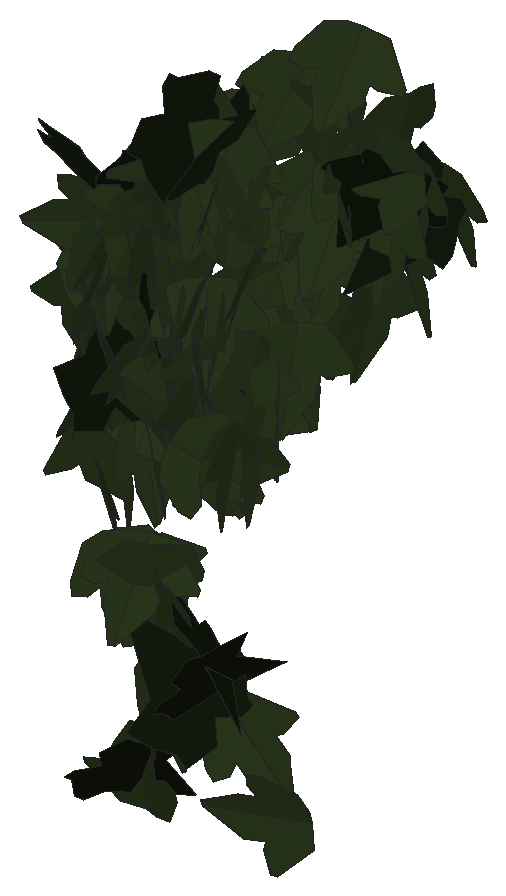
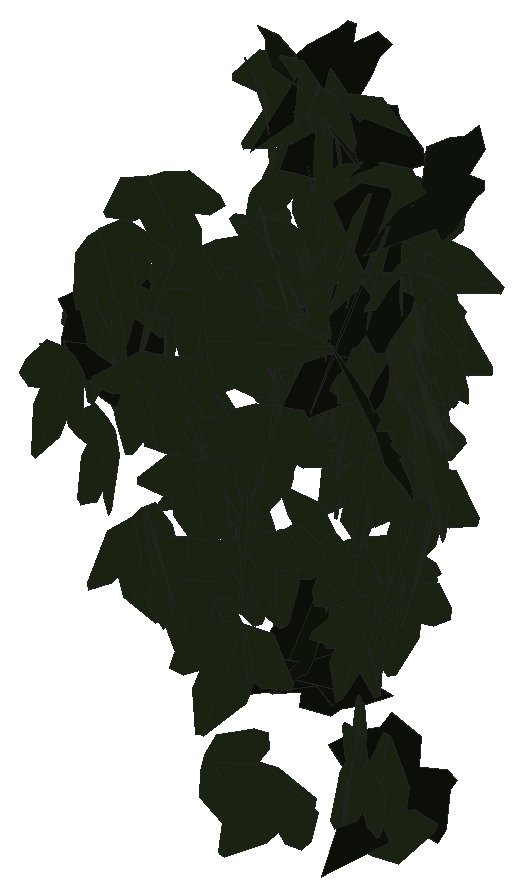
# SketchUp Ruby script. Lengths in inches.
U = 1.inch
M = Sketchup.active_model
def pt(a) = Geom::Point3d.new(a.map { |v| v * U })
def face(e, loops, mat)
  f = e.add_face(loops[0].map { |a| pt(a) })
  loops[1..].each { |l| e.add_face(l.map { |a| pt(a) }).erase! }
  f.material = f.back_material = mat if mat
  f
end
# faces: each face lists its corners as indices into pts; further lists are holes
def faces(e, pts, list, mat = nil) = list.each { |f| face(e, (f[0].is_a?(Array) ? f : [f]).map { |l| l.map { |i| pts[i] } }, mat) }
# xy, xz, yz: faces in a plane at the given z, y or x. An outline is a flat list of corners, or four numbers for a rectangle; further outlines are holes
def ring(l) = l.size == 4 ? [[l[0], l[1]], [l[2], l[1]], [l[2], l[3]], [l[0], l[3]]] : l.each_slice(2).to_a
def flat(e, list, mat, &to3) = list.each { |f| face(e, (f[0].is_a?(Array) ? f : [f]).map { |l| ring(l).map { |u, v| to3.(u, v) } }, mat) }
def xy(e, z, list, mat = nil) = flat(e, list, mat) { |x, y| [x, y, z] }
def xz(e, y, list, mat = nil) = flat(e, list, mat) { |x, z| [x, y, z] }
def yz(e, x, list, mat = nil) = flat(e, list, mat) { |y, z| [x, y, z] }
def lines(e, pts, list) = list.each { |a, b| e.add_line(pt(pts[a]), pt(pts[b])) }
# prism: a flat outline (further loops are holes) pulled along v
def prism(e, loops, v, mat = nil)
  f = face(e, loops, mat); d = Geom::Vector3d.new(v.map { |x| x * U })
  f.pushpull(f.normal.samedirection?(d) ? d.length : -d.length)
end
def box(e, o, s, mat = nil) = prism(e, [[o, [o[0] + s[0], o[1], o[2]], [o[0] + s[0], o[1] + s[1], o[2]], [o[0], o[1] + s[1], o[2]]]], [0, 0, s[2]], mat)
def at(x, y, z, deg = 0) = Geom::Transformation.translation(pt([x, y, z])) * Geom::Transformation.rotation(ORIGIN, Z_AXIS, deg.degrees)
def axes(o, x, y, z) = Geom::Transformation.new([*x, 0, *y, 0, *z, 0, *pt(o).to_a, 1])
def part(name) = M.definitions.add(name)
# library, detail: a bought-in or finely detailed component or shape, given as its bounding box
def library(name, o, s) = part(name).tap { |d| box(d.entities, o, s) }
def detail(e, o, s) = box(e.add_group.entities, o, s)
def put(e, d, t, mat = nil) = e.add_instance(d, t).tap { |i| i.material = mat if mat }
def group(e, t, mat = nil) = e.add_group.tap { |g| g.transformation = t; g.material = mat if mat }.entities
root = M.entities
M.materials.add("efeu1").color = [18, 25, 13]
M.materials.add("efeu2").color = [43, 57, 29]
c1 = part("ivyleaf_9")
p = [[1.54,2.16,1.25],[1.36,2.04,1.19],[-0.21,0.99,0.68],[-0.71,1.11,0.82],[-0.85,0.86,0.67],[-0.8,0.17,0.21],
  [-0.9,-0.01,0.1],[-0.67,-0.16,-0.02],[-0.08,-0.08,-0.05],[-0.03,-0.6,-0.4],[0.65,-0.88,-0.66],[0.83,-0.6,-0.49],
  [1.29,-0.42,-0.43],[1.8125,-0.07,-0.26],[1.21,0.44,0.15]]
faces(c1.entities,p,[[0,1,2,3,4,5,6,7,8,9,10,11,12,13,14]],"efeu1")
c2 = part("ivyleaf_10")
p = [[0,0.5,-0.03],[-0.0625,2.02,-0.43],[-0.19,2.01,-0.46],[-0.54,1.05,-0.29],[-0.52,0.625,-0.18],[-0.83,0.76,-0.28],
  [-1.16,0.64,-0.33],[-1.15,0.33,-0.24],[-0.77,-0.39,0.02],[-0.3,-0.51,0.16],[0.04,-0.48,0.23],[-0.02,2.01,-0.4375],
  [-0.06,2.01,-0.43],[0.04,-0.49,0.23],[0.67,-0.49,0.14],[1.38,0.36,-0.2],[1.375,0.51,-0.24],[0.81,0.65,-0.19],
  [0.62,0.59,-0.15],[0.6,1.09,-0.28],[0.5,1.23,-0.31]]
faces(c2.entities,p,[[0,1,2,3,4,5,6,7,8,9,10],[11,12,0,13,14,15,16,17,18,19,20]],"efeu2")
put(root,c1,axes([28.5,224.64,221.63],[0.47102,-0.15737,-0.05806],[-0.01733,0.12648,-0.48343],[0.16685,0.45742,0.1137]))
put(root,c2,axes([29.86,224.82,220.2],[0.40488,-0.28287,-0.07784],[-0.05263,0.06047,-0.49353],[0.28863,0.40783,0.01919]))
put(root,c2,axes([29.51,224.96,221.18],[-0.30399,-0.33355,0.21525],[-0.06846,-0.22299,-0.44225],[0.39103,-0.29835,0.0899]))
put(root,c2,axes([28.96,224.83,220.77],[0.15244,0.0172,-0.47589],[-0.47541,0.03413,-0.15105],[0.02729,0.49854,0.02676]))
put(root,c2,axes([30.44,224.62,219.81],[-0.21565,0.39061,0.22566],[-0.18174,0.15369,-0.43972],[-0.41288,-0.27167,0.07569]))
put(root,c2,axes([29.75,224.79,220.58],[-0.14398,0.47231,-0.07871],[0.02061,-0.07601,-0.49376],[-0.47838,-0.14542,0.00241]))
put(root,c2,axes([30.32,224.84,221.86],[-0.46236,0.14744,-0.12036],[0.08114,-0.13332,-0.47502],[-0.17217,-0.45879,0.09936]))
put(root,c1,axes([29.22,224.6875,218.73],[-0.21591,-0.302,0.33493],[0.19308,0.27368,0.37124],[-0.40756,0.28965,-0.00156]))
put(root,c2,axes([29.87,224.83,221.91],[-0.35993,-0.3449,-0.03865],[0.07684,-0.02489,-0.49343],[0.33845,-0.36114,0.07093]))
put(root,c2,axes([29.43,224.89,216.83],[0.38309,0.29352,-0.13072],[-0.09704,-0.08823,-0.48249],[-0.30631,0.39505,-0.01064]))
put(root,c1,axes([30.08,224.54,222.55],[0.15728,-0.13643,-0.45459],[-0.14102,0.44384,-0.18199],[0.45319,0.18546,0.10113]))
put(root,c2,axes([28.93,224.86,220.3],[0.2334,-0.44039,-0.03974],[-0.00565,0.04196,-0.4982],[0.44215,0.23301,0.01461]))
put(root,c2,axes([29.92,224.88,221.75],[-0.00922,-0.49985,-0.00831],[-0.00228,0.00835,-0.49993],[0.49991,-0.00918,-0.00243]))
put(root,c2,axes([29.28,224.93,219.24],[0.09109,-0.49047,0.0338],[0.00236,-0.03393,-0.49884],[0.49163,0.09103,-0.00387]))
put(root,c2,axes([30.38,224.92,221.83],[0.34542,0.33796,-0.12832],[-0.09579,-0.08556,-0.48322],[-0.34858,0.35842,0.00564]))
put(root,c2,axes([28.92,224.82,220.49],[0.07314,0.49378,-0.02883],[-0.01014,-0.02764,-0.49913],[-0.49452,0.0736,0.00597]))
put(root,c2,axes([30.56,224.875,222.22],[0.47817,0.1461,0.00346],[-0.00579,0.03077,-0.49902],[-0.14603,0.47719,0.03112]))
put(root,c1,axes([30.62,224.67,222.26],[-0.21297,0.40707,0.19732],[-0.17522,0.12684,-0.45079],[-0.41706,-0.26116,0.08863]))
put(root,c1,axes([29.24,224.53,214.37],[0.32817,0.34815,0.14525],[0.09195,0.11288,-0.47833],[-0.36586,0.34066,0.01006]))
put(root,c2,axes([30.58,224.99,218.59],[0.18188,-0.45439,0.10222],[0.10643,-0.06629,-0.48402],[0.45342,0.19783,0.07261]))
put(root,c2,axes([29.58,224.89,216.84],[-0.36258,-0.3396,0.0566],[-0.04507,-0.03466,-0.49676],[0.34132,-0.36533,-0.00548]))
put(root,c2,axes([29.05,224.73,219.42],[-0.35572,0.30882,0.16761],[-0.14985,0.0824,-0.46985],[-0.31782,-0.3845,0.03393]))
put(root,c2,axes([30.3,224.86,220.24],[0.42861,0.2521,0.05235],[0.03483,0.04396,-0.49684],[-0.25512,0.42955,0.02012]))
put(root,c2,axes([30.29,224.99,220.06],[0.40896,-0.25464,0.13382],[0.12416,-0.05356,-0.48137],[0.25948,0.42695,0.01942]))
put(root,c2,axes([28.87,225,220.33],[0.15952,-0.46639,0.08388],[0.04466,-0.07332,-0.49258],[0.47176,0.16464,0.01826]))
put(root,c2,axes([29.44,224.84,221.26],[-0.48057,-0.1347,0.0302],[-0.02883,-0.00905,-0.49909],[0.135,-0.48143,0.00093]))
put(root,c2,axes([30.36,225.02,219.4],[0.26041,-0.1776,-0.38813],[0.32126,-0.21781,0.3152],[-0.28104,-0.41354,0.00067]))
put(root,c2,axes([28.71,224.875,219.77],[-0.48333,-0.11894,0.04735],[-0.04415,-0.01871,-0.4977],[0.12016,-0.48529,0.00758]))
put(root,c1,axes([29.77,224.77,221.82],[0.18253,0.42089,-0.19883],[-0.08547,-0.17964,-0.45872],[-0.45758,0.20145,0.00637]))
put(root,c2,axes([30.37,224.96,221.7],[0.26776,-0.4187,-0.05477],[-0.02497,0.04904,-0.49696],[0.42152,0.26887,0.00535]))
put(root,c2,axes([30.3,224.625,218.47],[0.09526,0.29277,0.39396],[0.13006,0.37192,-0.30784],[-0.4733,0.16113,-0.00529]))
put(root,c2,axes([29.79,224.92,219.03],[-0.24499,0.42846,-0.07999],[0.00105,-0.09118,-0.49161],[-0.43587,-0.24105,0.04377]))
put(root,c1,axes([30.27,225.01,215.16],[-0.37535,-0.32362,-0.06625],[-0.0449,-0.04936,0.49553],[-0.32726,0.37794,0.00799]))
put(root,c2,axes([29.33,225.01,213.85],[-0.49988,0.00402,0.01023],[0.01019,-0.00493,0.49987],[0.00412,0.49996,0.00485]))
put(root,c2,axes([30.21,224.91,221.34],[-0.47942,-0.12458,0.06807],[-0.06848,-0.00704,-0.49524],[0.12436,-0.48418,-0.01031]))
put(root,c2,axes([28.68,224.99,218.59],[0.13114,-0.48104,-0.03747],[-0.00739,0.03682,-0.49859],[0.48244,0.13132,0.00255]))
put(root,c2,axes([30.47,224.98,219.66],[-0.23989,-0.43853,-0.01186],[0.00641,0.01002,-0.49986],[0.43865,-0.23997,0.00082]))
put(root,c1,axes([30.28,224.57,215.67],[0.21704,0.29037,0.34435],[0.18781,0.28909,-0.36215],[-0.40942,0.28655,0.01642]))
put(root,c2,axes([30.01,225.06,218.98],[0.08369,-0.4923,0.02514],[-0.00173,-0.02579,-0.49933],[0.49294,0.08349,-0.00602]))
put(root,c2,axes([28.92,225.04,219.82],[0.07813,-0.49384,0.00433],[0.00065,-0.00428,-0.49998],[0.49386,0.07813,-0.00002]))
put(root,c2,axes([29.57,224.9,221.23],[-0.29952,-0.35578,-0.18359],[0.13765,0.12378,-0.46447],[0.37595,-0.32878,0.0238]))
put(root,c1,axes([29.95,225.23,215.98],[0.20827,-0.38455,0.24238],[0.12913,-0.20557,-0.43711],[0.43583,0.24467,0.01369]))
put(root,c2,axes([28.49,225.04,219.85],[0.43149,-0.23739,0.0864],[0.12455,0.05112,-0.48153],[0.21979,0.43707,0.10325]))
put(root,c2,axes([28.51,225.2,219.41],[0.26146,-0.3783,0.19628],[0.11171,-0.1614,-0.45986],[0.41129,0.28432,0.00012]))
put(root,c2,axes([28.85,225.03,220.05],[0.26042,-0.41768,-0.08788],[-0.049,0.07301,-0.49221],[0.424,0.26498,-0.0029]))
put(root,c2,axes([28.71,224.93,220.2],[-0.48793,0.09989,0.04415],[-0.04199,0.01498,-0.49801],[-0.10082,-0.48969,-0.00622]))
put(root,c2,axes([29.93,225.07,219.88],[0.03164,-0.49898,-0.00439],[-0.01479,0.00346,-0.49977],[0.49878,0.03175,-0.01454]))
put(root,c2,axes([29.38,224.86,218.93],[-0.30313,-0.20771,-0.33907],[0.28343,0.18617,-0.36743],[0.27889,-0.41497,0.00488]))
put(root,c2,axes([29.86,224.92,220.4375],[-0.09439,0.48776,0.05641],[-0.00979,0.05556,-0.49681],[-0.49091,-0.09489,-0.00094]))
put(root,c2,axes([29.21,225.11,219.68],[-0.19374,-0.07213,0.45526],[-0.43067,-0.14767,-0.20667],[0.16427,-0.47222,-0.00491]))
put(root,c2,axes([28.78,225.17,219.78],[0.10086,-0.48315,0.07996],[0.00636,-0.08034,-0.49346],[0.48968,0.10056,-0.01006]))
put(root,c2,axes([29.7,225.08,218.61],[-0.29428,0.3865,-0.1184],[-0.00837,-0.15225,-0.47618],[-0.40414,-0.27828,0.09607]))
put(root,c2,axes([29.43,225.06,220.03],[-0.46218,0.06864,-0.17799],[0.16556,-0.08745,-0.46362],[-0.09477,-0.48749,0.05811]))
put(root,c2,axes([29.67,224.95,216.42],[-0.38508,0.05095,0.31483],[-0.30998,0.05631,-0.38825],[-0.07502,-0.4942,-0.01178]))
put(root,c2,axes([29.03,225.03,216.66],[0.3296,0.37326,0.04519],[0.03317,0.031,-0.49793],[-0.37452,0.33124,-0.00433]))
put(root,c2,axes([29.91,225.11,219.95],[-0.06857,0.48267,-0.11101],[-0.03777,-0.11684,-0.48469],[-0.49383,-0.05808,0.05248]))
put(root,c2,axes([30.12,225.09,220.25],[0.16913,-0.46492,-0.07241],[0.00618,0.07914,-0.49366],[0.47048,0.16609,0.03251]))
put(root,c2,axes([28.74,225.04,218.04],[-0.23927,-0.41112,-0.15404],[0.11309,0.1118,-0.47404],[0.42422,-0.26169,0.03948]))
put(root,c2,axes([29.55,225.09,219.23],[-0.37443,-0.08248,-0.32094],[0.32935,-0.03927,-0.37415],[0.03651,-0.49158,0.08374]))
put(root,c2,axes([30.81,224.95,218.48],[0.2715,-0.20375,-0.36711],[-0.234,0.28956,-0.33377],[0.34861,0.35305,0.06188]))
put(root,c2,axes([28.85,225.16,219.78],[0.1764,-0.46608,-0.04066],[0.00851,0.04665,-0.49775],[0.46777,0.17491,0.02439]))
put(root,c2,axes([30.59,225.2,220.58],[0.25408,-0.43038,-0.0146],[-0.00663,0.01303,-0.49979],[0.43058,0.25417,0.00092]))
put(root,c2,axes([29.5,225.09,218.4],[-0.46682,0.08312,-0.15864],[0.15513,-0.03365,-0.47413],[-0.0895,-0.49189,0.00562]))
put(root,c2,axes([29.8125,225.13,219.82],[0.00284,0.49529,-0.06838],[-0.00197,-0.06837,-0.4953],[-0.49999,0.00309,0.00156]))
put(root,c2,axes([30.79,224.99,221.58],[0.33346,-0.23364,0.2902],[-0.23353,0.17238,0.40713],[-0.29029,-0.40706,0.00584]))
put(root,c2,axes([29.94,225.21,222.32],[0.42954,-0.03928,0.25289],[0.25307,-0.00825,-0.43114],[0.03804,0.49839,0.0128]))
put(root,c2,axes([29.32,224.93,220.61],[-0.24853,0.355,0.24941],[-0.16654,0.18735,-0.43262],[-0.40062,-0.29811,0.02512]))
put(root,c1,axes([29.53,225,220.18],[0.2897,-0.2167,-0.34513],[-0.28088,0.20063,-0.36174],[0.29526,0.40347,-0.00549]))
put(root,c2,axes([30.2,225.03,220.02],[-0.24756,-0.23321,0.3665],[0.26601,0.25212,0.34011],[-0.34344,0.36338,-0.00075]))
put(root,c2,axes([28.72,225,220.24],[0.2607,0.25342,0.34324],[0.23085,0.2545,-0.36323],[-0.35881,0.34786,0.01569]))
put(root,c2,axes([29.38,225.13,218.25],[-0.25929,0.42745,-0.0076],[-0.02829,-0.02603,-0.49852],[-0.42658,-0.25809,0.03768]))
put(root,c2,axes([29.49,224.92,220.84],[0.03607,-0.29981,-0.39851],[0.03805,0.40004,-0.29752],[0.49724,-0.00887,0.05167]))
put(root,c2,axes([29.29,225.15,218.15],[0.08462,0.49278,0.0029],[-0.00095,0.00311,-0.49999],[-0.49279,0.08461,0.00146]))
put(root,c2,axes([28.71,225.08,219.23],[-0.08139,0.48587,0.08549],[-0.01965,0.08338,-0.49261],[-0.49294,-0.08354,0.00552]))
put(root,c2,axes([30.53,225.27,220.96],[-0.07968,0.4739,0.13808],[0.00292,-0.13941,0.48016],[0.4936,0.07732,0.01945]))
put(root,c2,axes([29.0625,225.23,219.56],[-0.21639,-0.44931,-0.03597],[0.05537,0.0131,-0.49675],[0.44734,-0.21897,0.04409]))
put(root,c2,axes([29.2,225.18,219.67],[0.00828,-0.05221,0.4972],[0.48415,0.12479,0.00504],[-0.12461,0.48135,0.05262]))
put(root,c2,axes([28.67,225.12,217.58],[-0.34313,0.3592,0.05692],[-0.04092,0.03962,-0.49675],[-0.36137,-0.34556,0.00221]))
put(root,c1,axes([29.125,225.45,219.99],[0.41525,-0.27357,0.05219],[-0.03328,0.04428,0.49692],[-0.27651,-0.41617,0.01857]))
put(root,c2,axes([29.68,225.11,218.61],[0.28965,-0.34572,-0.21583],[-0.01003,0.25866,-0.42778],[0.40743,0.25215,0.14291]))
put(root,c2,axes([29.3125,225.09,218.24],[0.46703,0.13716,-0.11431],[0.08607,0.10751,0.48066],[0.15643,-0.46865,0.07681]))
put(root,c2,axes([29.01,225.17,218.75],[-0.174,-0.43949,-0.163],[0.0487,0.15598,-0.47255],[0.46621,-0.18032,-0.01148]))
put(root,c2,axes([31.08,225.3,214.01],[0.04226,0.05638,-0.49501],[-0.49797,0.02028,-0.04021],[0.01554,0.4964,0.05786]))
put(root,c2,axes([29.52,225.09,215.07],[0.204,-0.33353,-0.31168],[-0.03673,0.32829,-0.37534],[0.45501,0.17603,0.10944]))
put(root,c2,axes([30.52,224.91,218.34],[0.07418,0.17336,0.46308],[-0.03427,0.46894,-0.17006],[-0.49328,-0.00651,0.08146]))
put(root,c1,axes([29.36,225.15,219.65],[0.49769,0.04701,0.00972],[0.00969,0.0008,-0.49991],[-0.04701,0.49778,-0.00011]))
put(root,c2,axes([28.95,225.21,219.36],[-0.34393,-0.2839,-0.22609],[0.17516,0.14295,-0.44596],[0.31785,-0.38596,0.00112]))
put(root,c2,axes([29.28,225.2,216.47],[0.07278,0.47115,0.15074],[0.00909,0.15106,-0.47655],[-0.49459,0.07211,0.01343]))
put(root,c2,axes([29.03,225.6,214.88],[0.34928,-0.21104,0.2889],[0.3228,0.01179,-0.38166],[0.15428,0.45313,0.14449]))
put(root,c2,axes([28.56,225.64,217.59],[-0.21896,0.4174,-0.16685],[0.04642,-0.1636,-0.47019],[-0.44711,-0.22139,0.03289]))
put(root,c1,axes([28.73,225.47,218.68],[-0.17382,0.41985,0.2086],[0.07848,-0.19328,0.45441],[0.4622,0.19071,0.00129]))
put(root,c2,axes([29.21,226.02,217.74],[0.33376,-0.00446,0.37227],[0.36802,0.07955,-0.32899],[-0.05629,0.49361,0.05639]))
put(root,c2,axes([29.87,225.97,214.44],[0.34481,0.15664,0.32645],[0.27837,0.1736,-0.37732],[-0.23155,0.44196,0.03251]))
put(root,c2,axes([30.01,226.04,218.63],[-0.00298,0.49783,-0.0464],[0.00169,-0.04639,-0.49784],[-0.49999,-0.00312,-0.0014]))
put(root,c2,axes([29.94,226.49,218.32],[0.35815,-0.33519,0.09682],[0.14525,0.01709,-0.47813],[0.31722,0.37061,0.10962]))
put(root,c2,axes([29.39,226.73,217.85],[0.30056,0.39251,-0.07486],[-0.06758,-0.04239,-0.4936],[-0.39382,0.30683,0.02757]))
put(root,c2,axes([29.92,226.87,218.67],[0.24408,0.4265,-0.09232],[-0.07299,-0.06438,-0.49043],[-0.43023,0.25289,0.03083]))
put(root,c2,axes([29.5,227.48,221.52],[0.39862,0.21923,-0.20746],[-0.21451,-0.03598,-0.45021],[-0.21233,0.44793,0.06537]))
put(root,c2,axes([30.2,227.5,222.12],[0.44094,0.19068,-0.1386],[-0.13369,-0.03986,-0.48014],[-0.19416,0.46049,0.01583]))
put(root,c2,axes([29.11,227.67,220.78],[0.00951,0.05354,0.49703],[-0.35573,-0.34856,0.04435],[0.35124,-0.35446,0.03146]))
put(root,c2,axes([30.79,227.58,220.78],[0.11108,-0.02581,-0.48682],[-0.48244,0.06594,-0.11357],[0.07006,0.49496,-0.01025]))
put(root,c2,axes([29.59,227.56,221.24],[-0.49323,-0.0779,0.02551],[-0.02599,0.00106,-0.49932],[0.07774,-0.49389,-0.00509]))
put(root,c1,axes([30.65,227.6,220.68],[0.14739,0.26586,-0.39698],[-0.25129,-0.31021,-0.30104],[-0.40636,0.28826,0.04217]))
put(root,c2,axes([28.7,227.6,219.89],[-0.41503,-0.27515,-0.04517],[0.03814,0.0242,-0.49796],[0.27621,-0.41678,0.0009]))
put(root,c2,axes([28.7,227.5625,219.91],[-0.28511,0.41074,-0.00017],[-0.00114,-0.00099,-0.5],[-0.41074,-0.28511,0.0015]))
put(root,c2,axes([29.55,227.87,220.18],[-0.1864,-0.38987,0.25151],[-0.01366,-0.26632,-0.42295],[0.46376,-0.16455,0.08863]))
put(root,c2,axes([29.29,227.6875,219.29],[0.42713,-0.12256,-0.22921],[-0.21918,0.06716,-0.44435],[0.13971,0.48007,0.00364]))
put(root,c2,axes([29.79,227.75,219.875],[0.45552,0.17259,-0.11277],[-0.10015,-0.05381,-0.4869],[-0.18021,0.46617,-0.01445]))
put(root,c2,axes([29.43,227.73,219.66],[0.46186,0.18726,-0.04027],[-0.03735,-0.01506,-0.49838],[-0.18787,0.46336,0.00008]))
put(root,c2,axes([29.83,227.8,220.59],[0.20356,-0.43497,0.13915],[0.21451,-0.04343,-0.44955],[0.40317,0.24272,0.16893]))
put(root,c2,axes([30.48,227.81,220.05],[0.48577,-0.10552,0.05376],[0.05107,-0.01811,-0.49705],[0.10685,0.4884,-0.00682]))
put(root,c2,axes([30.03,227.68,221.23],[-0.29041,0.40598,-0.02905],[0.02117,-0.02057,-0.49913],[-0.40647,-0.29113,-0.00524]))
put(root,c2,axes([30.63,227.83,221.39],[-0.08301,-0.49043,0.05084],[-0.00417,-0.05086,-0.49739],[0.49304,-0.083,0.00435]))
put(root,c2,axes([29.4,227.82,219.2],[0.45775,0.20049,0.01657],[0.00329,0.0337,-0.49885],[-0.20114,0.4568,0.02954]))
put(root,c2,axes([30.68,227.875,220.68],[-0.4652,0.18321,0.00536],[-0.02951,-0.06045,-0.49545],[-0.18089,-0.46128,0.06705]))
put(root,c2,axes([28.67,227.94,218.625],[0.32374,0.37878,-0.04147],[-0.01923,-0.03811,-0.49817],[-0.38055,0.32416,-0.01011]))
put(root,c1,axes([30.8,228.13,220.23],[-0.49634,-0.05892,-0.01341],[0.01329,0.00187,-0.49982],[0.05894,-0.49651,-0.00029]))
put(root,c2,axes([29.17,227.9,218.01],[0.3749,-0.13198,-0.30336],[-0.2527,0.18167,-0.39133],[0.21352,0.44674,0.06951]))
put(root,c2,axes([28.71,227.86,219.04],[0.13499,-0.41662,-0.24126],[-0.01245,0.24746,-0.43429],[0.48127,0.12326,0.05643]))
put(root,c2,axes([29.81,227.96,220.33],[0.24156,0.40601,0.16373],[0.06428,0.15208,-0.47195],[-0.43303,0.24906,0.02128]))
put(root,c2,axes([28.71,228.14,217.58],[-0.36654,-0.30615,-0.14806],[0.15368,0.04507,-0.47366],[0.30337,-0.39273,0.06106]))
put(root,c2,axes([29.33,228.19,218.38],[-0.48028,-0.12064,0.0691],[-0.06488,-0.02531,-0.49513],[0.12296,-0.48457,0.00865]))
put(root,c2,axes([30.31,228.28,219.46],[-0.37137,0.25965,-0.21134],[0.13988,-0.16642,-0.45026],[-0.30416,-0.39356,0.05097]))
put(root,c2,axes([29.49,228.29,218.04],[0.29287,-0.40136,0.05603],[-0.04059,0.03972,0.49676],[-0.40321,-0.29552,-0.00932]))
put(root,c2,axes([29.84,228.35,218.58],[0.05055,0.49292,-0.0669],[-0.18418,-0.04392,-0.46276],[-0.46209,0.07142,0.17713]))
put(root,c2,axes([30.67,228.51,220.24],[-0.44811,0.208,-0.07704],[0.06811,-0.03625,-0.49401],[-0.2111,-0.45323,0.00415]))
